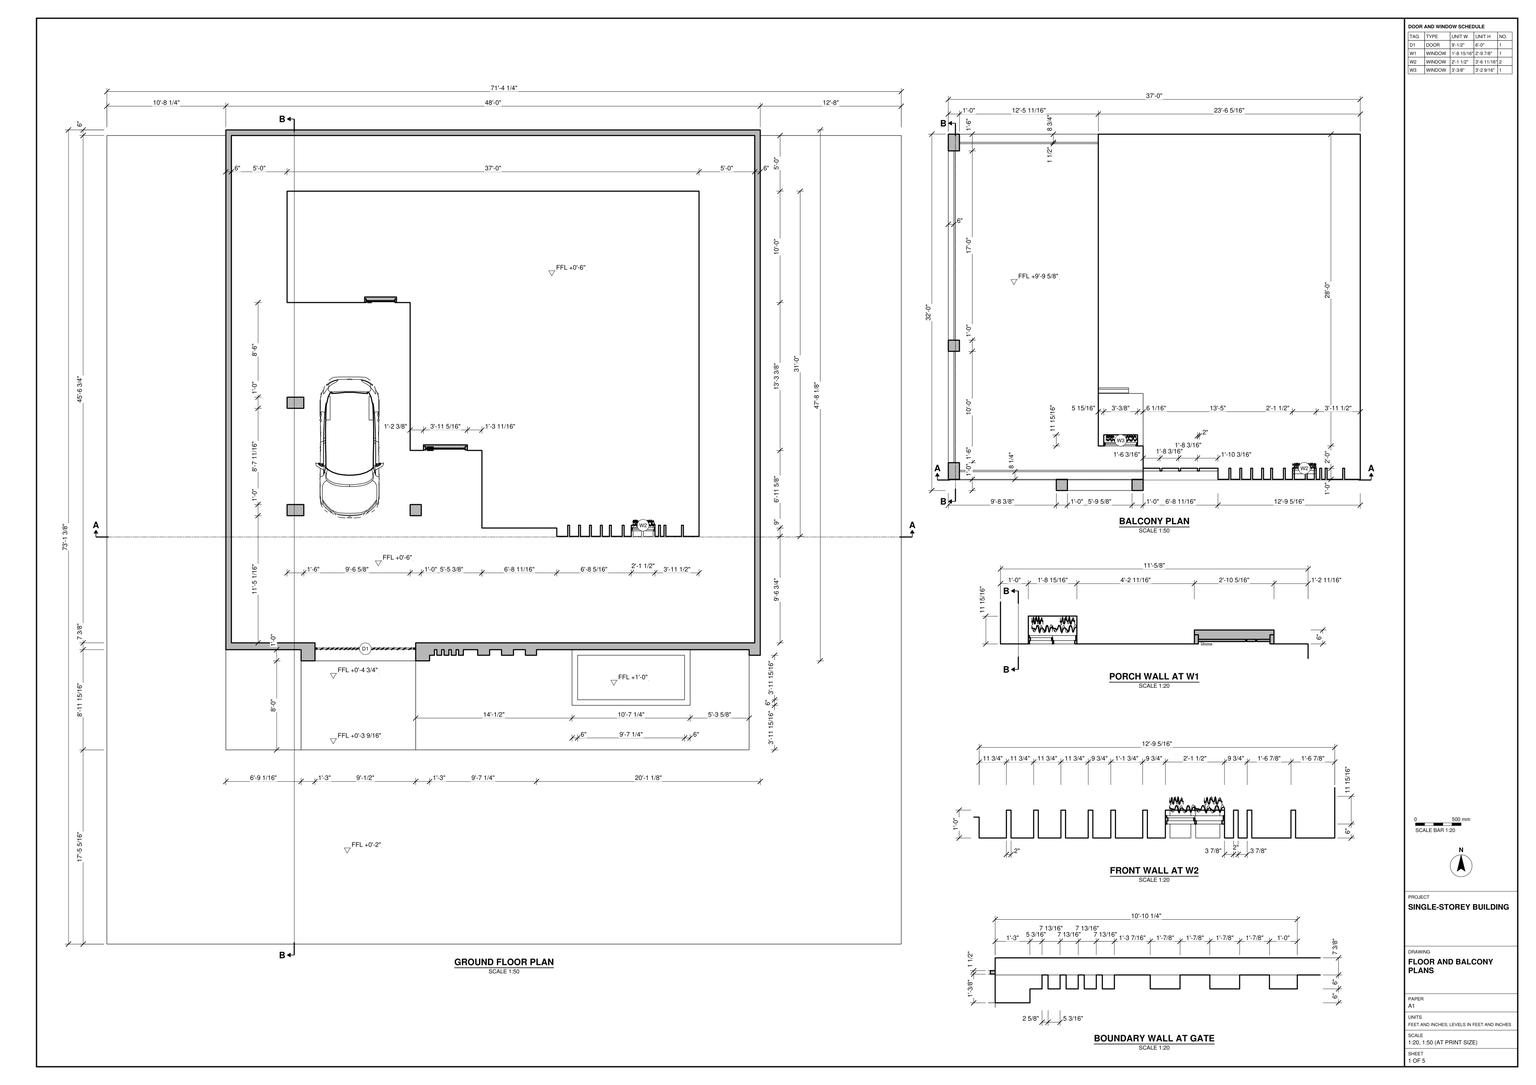
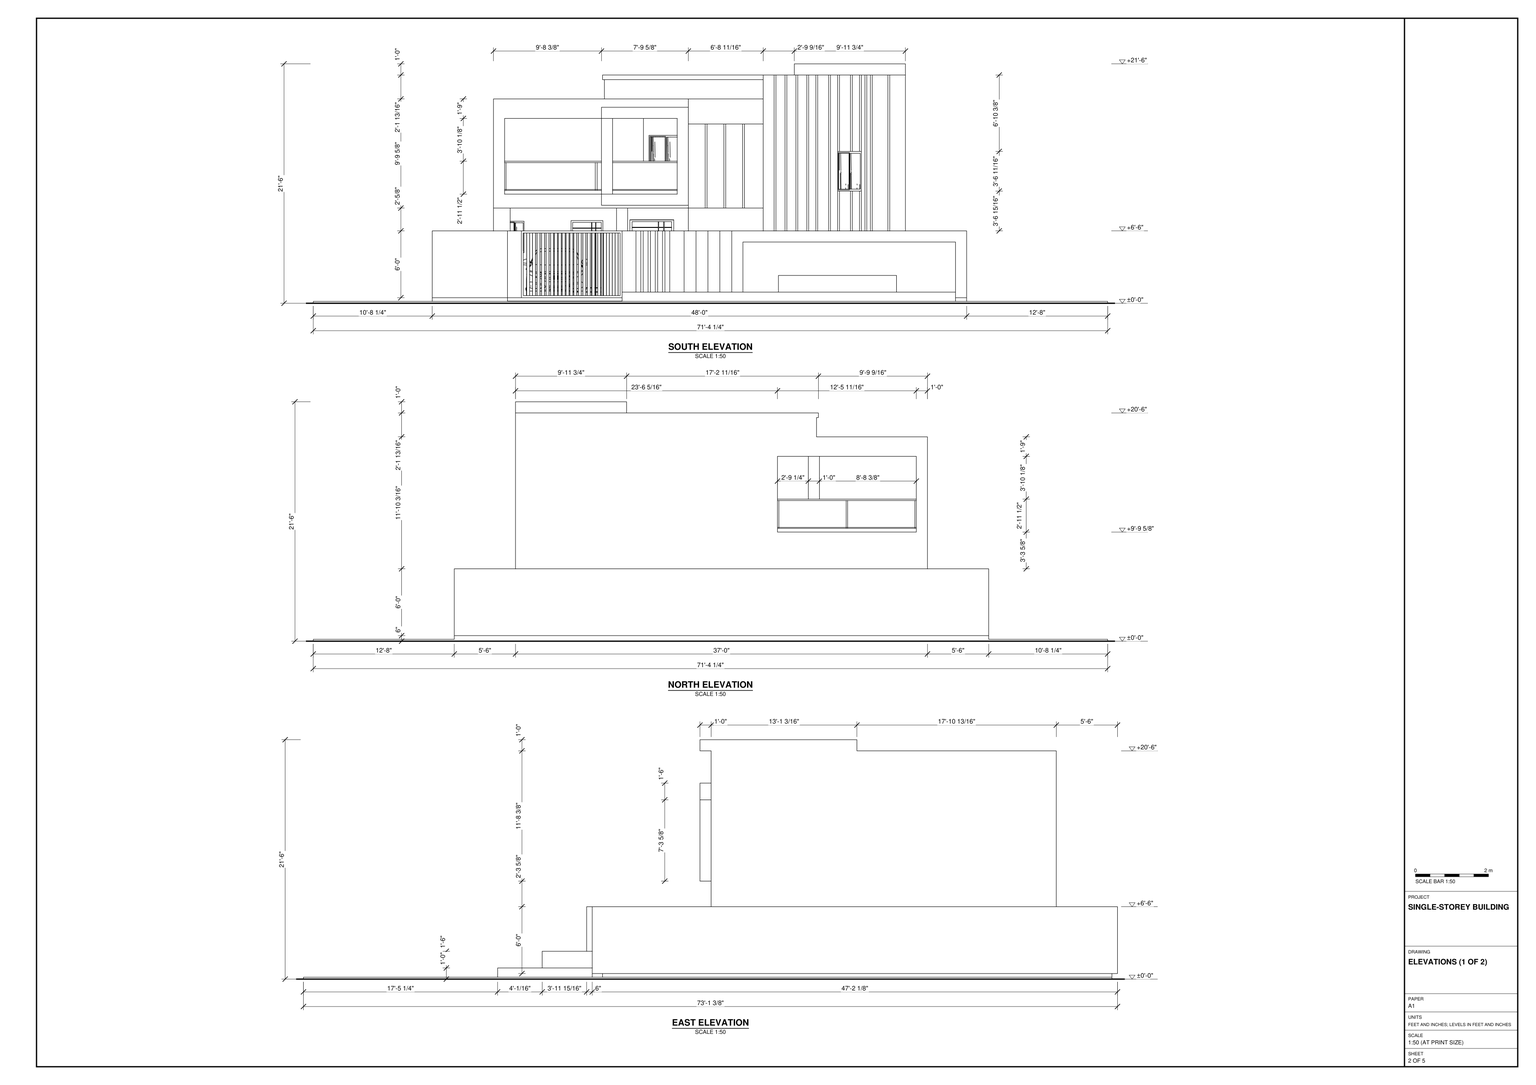
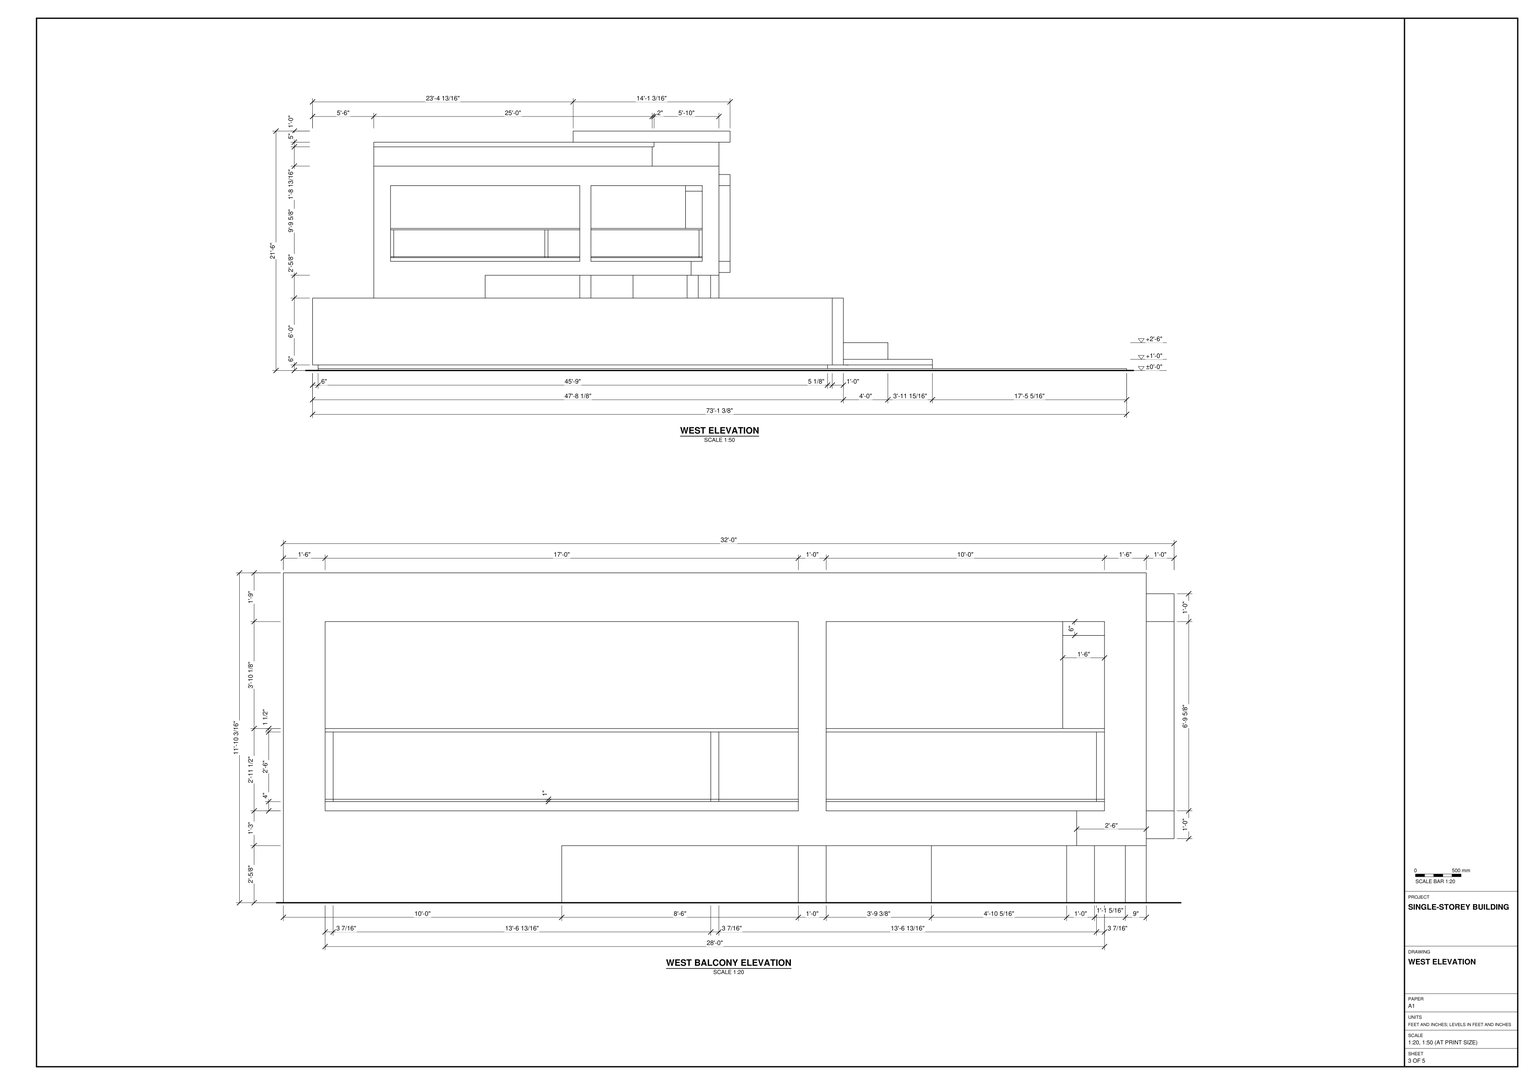
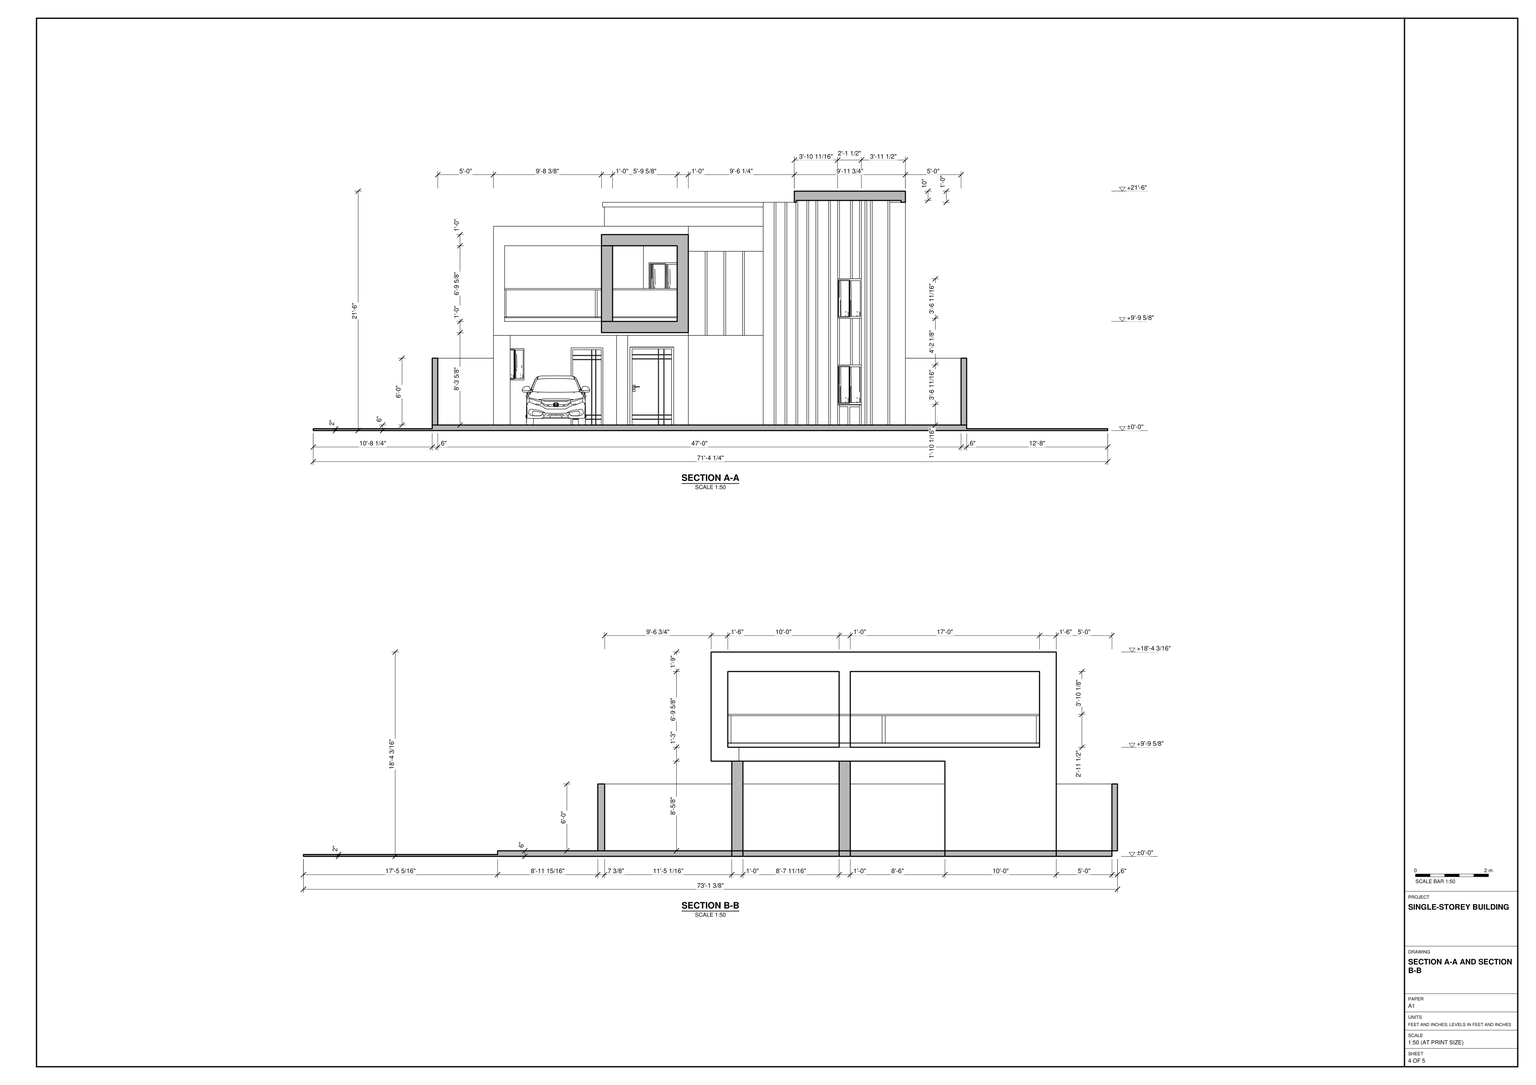
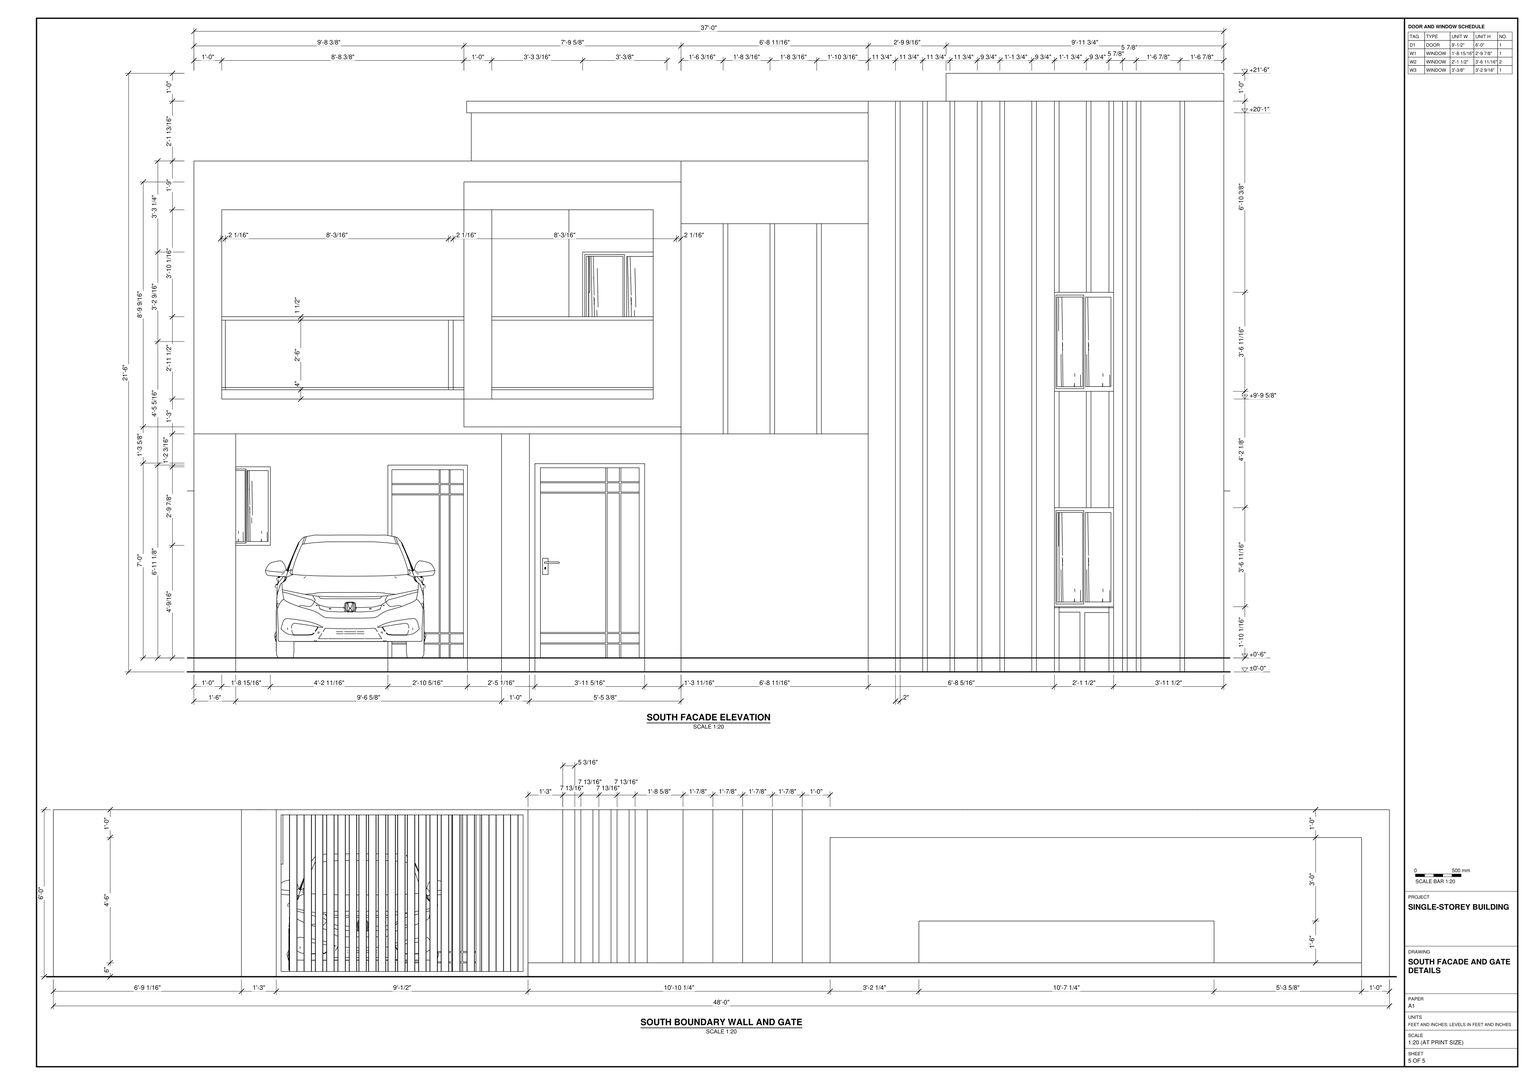
Build the house and its site in SketchUp from task_files/diagram_01.pdf. Work in feet and inches. Use ±0'-0" as the ground-floor datum. The complete model, including the site base, must measure 71'-4 1/4" east to west, 73'-1 3/8" north to south and 21'-6" high.

Lay out the boundary walls inside the site base, leaving the approach in front of the south gate. Follow the wall thicknesses in plan, including the 6" side boundary walls. Model the barred gate, the changing profile of the wall beside it and the low rectangular feature in front of the wall. Set the house back from the enclosure and follow the stepped ground-floor outline to form the recessed parking porch. Place the car under the balcony, in line with the gate.

Use the balcony plan and elevations to position the slab, supports, rectangular balcony frames and glass railing panels. Match the scheduled openings, the vertical fins around the front window and the stepped flat roof profile. Keep walls, slabs, roof elements and each furniture or joinery piece in separate groups or components, and use components for repeated parts. Decor and loose items, including the car, may be any suitable library components. Save one SketchUp model as output_files/single_storey_house_with_framed_balcony_and_gated_yard.skp.

# SketchUp Ruby script. Lengths in inches.
U = 1.inch
M = Sketchup.active_model
def pt(a) = Geom::Point3d.new(a.map { |v| v * U })
def face(e, loops, mat)
  f = e.add_face(loops[0].map { |a| pt(a) })
  loops[1..].each { |l| e.add_face(l.map { |a| pt(a) }).erase! }
  f.material = f.back_material = mat if mat
  f
end
# faces: each face lists its corners as indices into pts; further lists are holes
def faces(e, pts, list, mat = nil) = list.each { |f| face(e, (f[0].is_a?(Array) ? f : [f]).map { |l| l.map { |i| pts[i] } }, mat) }
# xy, xz, yz: faces in a plane at the given z, y or x. An outline is a flat list of corners, or four numbers for a rectangle; further outlines are holes
def ring(l) = l.size == 4 ? [[l[0], l[1]], [l[2], l[1]], [l[2], l[3]], [l[0], l[3]]] : l.each_slice(2).to_a
def flat(e, list, mat, &to3) = list.each { |f| face(e, (f[0].is_a?(Array) ? f : [f]).map { |l| ring(l).map { |u, v| to3.(u, v) } }, mat) }
def xy(e, z, list, mat = nil) = flat(e, list, mat) { |x, y| [x, y, z] }
def xz(e, y, list, mat = nil) = flat(e, list, mat) { |x, z| [x, y, z] }
def yz(e, x, list, mat = nil) = flat(e, list, mat) { |y, z| [x, y, z] }
def lines(e, pts, list) = list.each { |a, b| e.add_line(pt(pts[a]), pt(pts[b])) }
# prism: a flat outline (further loops are holes) pulled along v
def prism(e, loops, v, mat = nil)
  f = face(e, loops, mat); d = Geom::Vector3d.new(v.map { |x| x * U })
  f.pushpull(f.normal.samedirection?(d) ? d.length : -d.length)
end
def box(e, o, s, mat = nil) = prism(e, [[o, [o[0] + s[0], o[1], o[2]], [o[0] + s[0], o[1] + s[1], o[2]], [o[0], o[1] + s[1], o[2]]]], [0, 0, s[2]], mat)
def at(x, y, z, deg = 0) = Geom::Transformation.translation(pt([x, y, z])) * Geom::Transformation.rotation(ORIGIN, Z_AXIS, deg.degrees)
def axes(o, x, y, z) = Geom::Transformation.new([*x, 0, *y, 0, *z, 0, *pt(o).to_a, 1])
def part(name) = M.definitions.add(name)
# library, detail: a bought-in or finely detailed component or shape, given as its bounding box
def library(name, o, s) = part(name).tap { |d| box(d.entities, o, s) }
def detail(e, o, s) = box(e.add_group.entities, o, s)
def put(e, d, t, mat = nil) = e.add_instance(d, t).tap { |i| i.material = mat if mat }
def group(e, t, mat = nil) = e.add_group.tap { |g| g.transformation = t; g.material = mat if mat }.entities
root = M.entities
M.materials.add("Glass Railing Color").color = [198, 198, 198]
M.materials.add("Railing Glass").color = [63, 150, 137]
M.materials["Railing Glass"].alpha = 0.13
M.materials.add("[0053_Ivory]").color = [239, 239, 225]
M.materials.add("[0053_Ivory]1").color = [249, 249, 235]
M.materials.add("[0132_LightGray]").color = [169, 169, 169]
M.materials.add("[0135_DarkGray]").color = [81, 81, 81]
M.materials.add("[0136_Charcoal]").color = [48, 48, 48]
M.materials.add("[Concrete Block 8x8 Gray]").color = [210, 211, 206]
M.materials.add("[Stone Sandstone Ashlar Light]").color = [206, 178, 128]
M.materials.add("[Wood Veneer 01]").color = [120, 70, 37]
c1 = library("window",[15.03,5.78,0],[94.49,11.94,82.51])
c2 = part("Glass Rail Spacer")
box(c2.entities,[-0.5,-0.25,0],[1,0.5,1],"Glass Railing Color")
c3 = part("Group138\#1")
prism(c3.entities,[[[0.54,0,1.27],[0.38,0,1.39],[0.21,0,1.47],[0.01,0,1.5],[-0.18,0,1.48],[-0.37,0,1.41],[-0.52,0,1.29],[-0.64,0,1.13],[-0.72,0,0.96],[-0.75,0,0.76],[-0.73,0,0.57],[-0.66,0,0.38],[-0.54,0,0.23],[-0.38,0,0.11],[-0.21,0,0.03],[-0.01,0,0],[0.18,0,0.02],[0.37,0,0.09],[0.52,0,0.21],[0.64,0,0.37],[0.72,0,0.54],[0.75,0,0.74],[0.73,0,0.93],[0.66,0,1.12]]],[0,97,0],"Glass Railing Color")
c4 = part("Group141\#1")
prism(c4.entities,[[[0.25,0,5],[0.25,0,4],[-0.25,0,4],[-0.25,0,5],[-0.5,0,5],[-0.5,0,0],[0.5,0,0],[0.5,0,5]]],[0,97,0],"Glass Railing Color")
c5 = part("Group144\#1")
box(c5.entities,[-0.1875,0,0],[0.375,47,30],"Railing Glass")
c6 = part("Group147\#1")
box(c6.entities,[-0.1875,0,0],[0.375,47,30],"Railing Glass")
c7 = part("Glass Railing\#8")
put(c7.entities,c2,at(0,0,4))
put(c7.entities,c2,at(48,0,4))
put(c7.entities,c2,at(96,0,4))
put(c7.entities,c3,at(-0.5,0,34,-90))
put(c7.entities,c4,at(-0.5,0,0,-90))
put(c7.entities,c5,at(0.5,0,4,-90))
put(c7.entities,c6,at(48.5,0,4,-90))
c8 = library("Untitled (9)",[0,0,0],[36,4.39,84])
c9 = part("Group\#2")
box(c9.entities,[0,-0.5,0],[45,3,0.125])
c10 = part("Wade+gate+4.0")
p = [[1.5,-0.75,79.5],[1.5,-0.75,82.5]]
lines(c10.entities,p,[[0,1]])
g1 = group(c10.entities,at(0,-1.5,0),"[Wood Veneer 01]")
prism(g1,[[[48,0,6],[48,0,84],[0,0,84],[0,0,6]],[[46.5,0,82.5],[46.5,0,7.5],[1.5,0,7.5],[1.5,0,82.5]]],[0,1.5,0])
put(c10.entities,c9,axes([1.5,-1.46,78.96],[1,0,0],[0,0.64279,0.76604],[0,-0.76604,0.64279]),"[Wood Veneer 01]")
put(c10.entities,c9,axes([1.5,-1.46,74.46],[1,0,0],[0,0.64279,0.76604],[0,-0.76604,0.64279]),"[Wood Veneer 01]")
put(c10.entities,c9,axes([1.5,-1.46,69.96],[1,0,0],[0,0.64279,0.76604],[0,-0.76604,0.64279]),"[Wood Veneer 01]")
put(c10.entities,c9,axes([1.5,-1.46,65.46],[1,0,0],[0,0.64279,0.76604],[0,-0.76604,0.64279]),"[Wood Veneer 01]")
put(c10.entities,c9,axes([1.5,-1.46,60.96],[1,0,0],[0,0.64279,0.76604],[0,-0.76604,0.64279]),"[Wood Veneer 01]")
put(c10.entities,c9,axes([1.5,-1.46,57.46],[1,0,0],[0,0.64279,0.76604],[0,-0.76604,0.64279]),"[Wood Veneer 01]")
put(c10.entities,c9,axes([1.5,-1.46,53.96],[1,0,0],[0,0.64279,0.76604],[0,-0.76604,0.64279]),"[Wood Veneer 01]")
put(c10.entities,c9,axes([1.5,-1.46,50.46],[1,0,0],[0,0.64279,0.76604],[0,-0.76604,0.64279]),"[Wood Veneer 01]")
put(c10.entities,c9,axes([1.5,-1.46,46.96],[1,0,0],[0,0.64279,0.76604],[0,-0.76604,0.64279]),"[Wood Veneer 01]")
put(c10.entities,c9,axes([1.5,-1.46,43.96],[1,0,0],[0,0.64279,0.76604],[0,-0.76604,0.64279]),"[Wood Veneer 01]")
put(c10.entities,c9,axes([1.5,-1.46,40.96],[1,0,0],[0,0.64279,0.76604],[0,-0.76604,0.64279]),"[Wood Veneer 01]")
put(c10.entities,c9,axes([1.5,-1.46,37.96],[1,0,0],[0,0.64279,0.76604],[0,-0.76604,0.64279]),"[Wood Veneer 01]")
put(c10.entities,c9,axes([1.5,-1.46,34.96],[1,0,0],[0,0.64279,0.76604],[0,-0.76604,0.64279]),"[Wood Veneer 01]")
put(c10.entities,c9,axes([1.5,-1.46,31.96],[1,0,0],[0,0.64279,0.76604],[0,-0.76604,0.64279]),"[Wood Veneer 01]")
put(c10.entities,c9,axes([1.5,-1.46,28.96],[1,0,0],[0,0.64279,0.76604],[0,-0.76604,0.64279]),"[Wood Veneer 01]")
put(c10.entities,c9,axes([1.5,-1.46,25.46],[1,0,0],[0,0.64279,0.76604],[0,-0.76604,0.64279]),"[Wood Veneer 01]")
put(c10.entities,c9,axes([1.5,-1.46,21.96],[1,0,0],[0,0.64279,0.76604],[0,-0.76604,0.64279]),"[Wood Veneer 01]")
put(c10.entities,c9,axes([1.5,-1.46,18.46],[1,0,0],[0,0.64279,0.76604],[0,-0.76604,0.64279]),"[Wood Veneer 01]")
put(c10.entities,c9,axes([1.5,-1.46,14.96],[1,0,0],[0,0.64279,0.76604],[0,-0.76604,0.64279]),"[Wood Veneer 01]")
put(c10.entities,c9,axes([1.5,-1.46,10.46],[1,0,0],[0,0.64279,0.76604],[0,-0.76604,0.64279]),"[Wood Veneer 01]")
c11 = library("car\#1",[0.01,0.03,0.02],[18.76,39.97,12.32])
xy(root,-6,[[[0,0,856.25,871.375],[484.9375,439.375,484.9375,448.375,404.25,448.375,404.25,532,388.57,532,388.57,538,341.26,538,341.26,532,326.88,532,326.88,691.375,312.17,691.375,312.17,697.375,277.86,697.375,277.86,691.375,194.25,691.375,194.25,811.375,638.25,811.375,638.25,439.375,621.37,439.375,621.37,451.375,619.37,451.375,619.37,439.375,602.49,439.375,602.49,451.375,600.49,451.375,600.49,439.375,596.62,439.375,596.62,451.375,594.62,451.375,594.62,439.375,590.74,439.375,590.74,451.375,588.74,451.375,588.74,439.375,578.3,439.375,578.3,451.375,576.23,451.375,576.23,439.375,567.23,439.375,567.23,451.375,565.23,451.375,565.23,439.375,557.47,439.375,557.47,451.375,555.47,451.375,555.47,439.375,543.72,439.375,543.72,451.375,541.72,451.375,541.72,439.375,533.96,439.375,533.96,451.375,531.96,451.375,531.96,439.375,522.2,439.375,522.2,451.375,520.2,451.375,520.2,439.375,510.45,439.375,510.45,451.375,508.45,451.375,508.45,439.375,498.69,439.375,498.69,451.375,496.69,451.375,496.69,439.375],[194.25,461.6875,212.25,473.6875],[194.25,577.375,212.25,589.375],[326.88,461.6875,338.88,473.6875]],[484.9375,439.375,496.69,439.375,496.69,451.375,498.69,451.375,498.69,439.375,508.45,439.375,508.45,451.375,510.45,451.375,510.45,439.375,520.2,439.375,520.2,451.375,522.2,451.375,522.2,439.375,531.96,439.375,531.96,451.375,533.96,451.375,533.96,439.375,541.72,439.375,541.72,451.375,543.72,451.375,543.72,439.375,555.47,439.375,555.47,451.375,557.47,451.375,557.47,439.375,565.23,439.375,565.23,451.375,567.23,451.375,567.23,439.375,576.23,439.375,576.23,451.375,578.3,451.375,578.3,439.375,588.74,439.375,588.74,451.375,590.74,451.375,590.74,439.375,594.62,439.375,594.62,451.375,596.62,451.375,596.62,439.375,600.49,439.375,600.49,451.375,602.49,451.375,602.49,439.375,619.37,439.375,619.37,451.375,621.37,451.375,621.37,439.375,638.25,439.375,638.25,461.6875,404.25,461.6875,404.25,448.375,484.9375,448.375],[194.25,461.6875,212.25,473.6875],[404.25,461.6875,638.25,461.6875,638.25,811.375,194.25,811.375,194.25,691.375,277.86,691.375,277.86,697.375,312.17,697.375,312.17,691.375,326.88,691.375,326.88,532,341.26,532,341.26,538,388.57,538,388.57,532,404.25,532],[326.88,461.6875,338.88,473.6875],
  [194.25,577.375,212.25,589.375]])
xy(root,-4,[[209.36,209.28,332.875,209.3125,332.85,305.25,209.33,305.22],[332.875,209.3125,332.875,305.25,332.85,305.25]])
xy(root,-4,[[0,0,856.25,0,856.25,871.375,704.25,871.375,704.25,311.25,692.25,311.25,692.25,209.3125,332.875,209.3125,209.36,209.28,209.33,305.22,332.85,305.25,209.33,305.25,209.33,209.28,128.25,209.28,128.25,871.375,0,871.375]],"[Concrete Block 8x8 Gray]")
xy(root,0,[[209.33,305.25,209.33,317.25,128.25,317.25,128.25,322.375,134.25,322.375,134.25,324.625,224.33,324.625,224.33,305.25],[[224.33,305.25,332.85,305.25,332.85,324.625,698.25,324.625,698.25,871.375,134.25,871.375,134.25,324.625,224.33,324.625],[194.25,577.375,212.25,589.375],[194.25,461.6875,212.25,473.6875],[326.88,461.6875,338.88,473.6875]],[332.85,305.25,332.875,317.25],[332.875,305.25,332.875,317.25,353.05,317.25,353.05,311.25,347.85,311.25,347.85,305.25],[692.25,311.25,692.25,317.25,332.85,317.25,332.85,324.625,698.25,324.625,698.25,322.375,704.25,322.375,704.25,311.25],
  [355.65,311.25,360.85,317.25],[363.45,311.25,368.65,317.25],[371.25,311.25,376.45,317.25],[379.05,311.25,384.25,317.25],[399.7,311.25,412.55,317.25],
  [425.4,311.25,438.25,317.25],[451.1,311.25,463.1,317.25],[128.25,322.375,134.25,871.375],[698.25,322.375,704.25,871.375],[128.25,871.375,704.25,877.375]])
xy(root,0,[[194.25,461.6875,212.25,473.6875],[326.88,461.6875,338.88,473.6875],[194.25,577.375,212.25,589.375]],"[0135_DarkGray]")
xy(root,0,[[128.25,209.28,209.33,317.25]],"[Concrete Block 8x8 Gray]")
xy(root,6,[[507.39,263.28,622.64,311.25]],"[0053_Ivory]1")
xy(root,6,[[332.875,209.3125,692.25,209.3125,692.25,317.25,628.64,317.25,628.64,257.28,501.39,257.28,501.39,317.25,463.1,317.25,463.1,311.25,451.1,311.25,451.1,317.25,438.25,317.25,438.25,311.25,425.4,311.25,425.4,317.25,412.55,317.25,412.55,311.25,399.7,311.25,399.7,317.25,384.25,317.25,384.25,311.25,379.05,311.25,379.05,317.25,376.45,317.25,376.45,311.25,371.25,311.25,371.25,317.25,368.65,317.25,368.65,311.25,363.45,311.25,363.45,317.25,360.85,317.25,360.85,311.25,355.65,311.25,355.65,317.25,353.05,317.25,353.05,311.25,347.85,311.25,347.85,305.25,332.875,305.25]],"[Concrete Block 8x8 Gray]")
xy(root,19.5625,[[578.3,439.375,588.74,451.375]],"[Wood Veneer 01]")
xy(root,19.75,[[567.23,439.375,576.23,451.375]],"[Wood Veneer 01]")
xy(root,24,[[[501.39,257.28,628.64,317.25],[507.39,263.28,622.64,311.25]]],"[0053_Ivory]1")
xy(root,48.54,[[206.26,691.375,227.2,703.375]])
xy(root,60,[[463.1,311.25,692.25,317.25]],"[0135_DarkGray]")
xy(root,64.77,[[567.23,439.375,578.98,451.375]],"[0135_DarkGray]")
xy(root,64.77,[[580.98,439.375,588.74,451.375]],"[Wood Veneer 01]")
xy(root,72,[[209.33,305.25,224.33,305.25,224.33,324.625,134.25,324.625,134.25,871.375,698.25,871.375,698.25,324.625,332.85,324.625,332.85,305.25,347.85,305.25,347.85,311.25,353.05,311.25,353.05,317.25,355.65,317.25,355.65,311.25,360.85,311.25,360.85,317.25,363.45,317.25,363.45,311.25,368.65,311.25,368.65,317.25,371.25,317.25,371.25,311.25,376.45,311.25,376.45,317.25,379.05,317.25,379.05,311.25,384.25,311.25,384.25,317.25,399.7,317.25,399.7,311.25,412.55,311.25,412.55,317.25,425.4,317.25,425.4,311.25,438.25,311.25,438.25,317.25,451.1,317.25,451.1,311.25,704.25,311.25,704.25,877.375,128.25,877.375,128.25,317.25,209.33,317.25]],"[0053_Ivory]1")
xy(root,82.42,[[206.26,691.375,227.2,703.375]])
xy(root,83.125,[[277.86,691.375,312.17,697.375]])
xy(root,83.75,[[341.26,532,388.57,538]])
xy(root,96.6,[[404.25,448.375,422.42,451.375],[424.42,448.375,442.59,451.375],[444.59,448.375,462.77,451.375],[464.77,448.375,484.9375,451.375],[194.25,461.6875,212.25,473.6875],
  [194.25,577.375,212.25,589.375]])
xy(root,96.6,[[[194.25,439.375,194.25,461.6875,212.25,461.6875,212.25,473.6875,194.25,473.6875,194.25,577.375,212.25,577.375,212.25,589.375,194.25,589.375,194.25,691.375,326.88,691.375,326.88,532,404.25,532,404.25,439.375],[326.88,461.6875,338.88,473.6875]]],"[0053_Ivory]")
xy(root,99.6,[[310.65,427.375,404.25,439.375]],"[0135_DarkGray]")
xy(root,111.6,[[310.65,427.375,322.65,439.375]])
xy(root,111.6,[[206.25,439.375,404.25,439.375,404.25,475.375,355.91,475.375,355.91,811.375,206.25,811.375,206.25,793.375,194.25,793.375,194.25,589.375,206.25,589.375,206.25,577.375,194.25,577.375,194.25,457.375,206.25,457.375]],"[0053_Ivory]")
xy(root,111.6,[[322.65,427.375,392.25,439.375]],"[0135_DarkGray]")
xy(root,114.91,[[567.23,439.375,578.98,451.375]],"[0135_DarkGray]")
xy(root,114.91,[[580.98,439.375,588.74,451.375]],"[Wood Veneer 01]")
xy(root,136.41,[[361.82,475.375,398.19,487.375]])
xy(root,157.61,[[567.23,439.375,578.98,451.375]],"[0135_DarkGray]")
xy(root,157.61,[[580.98,439.375,588.74,451.375]],"[Wood Veneer 01]")
xy(root,174.97,[[361.82,475.375,398.19,487.375]])
xy(root,187.2,[[404.25,439.375,404.25,451.375,422.42,451.375,422.42,448.375,424.42,448.375,424.42,451.375,442.59,451.375,442.59,448.375,444.59,448.375,444.59,451.375,462.77,451.375,462.77,448.375,464.77,448.375,464.77,451.375,484.9375,451.375,484.9375,439.375]],"[0053_Ivory]")
xy(root,193.2,[[310.65,427.375,322.65,439.375]])
xy(root,193.2,[[[206.25,439.375,206.25,457.375,194.25,457.375,194.25,577.375,206.25,577.375,206.25,589.375,194.25,589.375,194.25,793.375,206.25,793.375,206.25,811.375,355.91,811.375,355.91,475.375,404.25,475.375,404.25,439.375],[206.46,481.3125,293.09,508.1875],[206.46,517.27,293.09,544.14],[206.46,553.22,293.09,580.1],[206.46,589.18,293.09,616.05],[206.46,625.13,293.09,652.01],[206.46,661.09,293.09,687.96],[206.46,733,293.09,759.875],[206.46,697.04,293.09,723.92]]],"[0053_Ivory]")
xy(root,193.2,[[322.65,427.375,392.25,439.375]],"[0135_DarkGray]")
xy(root,205.2,[[310.65,427.375,404.25,439.375]],"[0136_Charcoal]")
xy(root,214.2,[[[194.25,439.375,484.9375,439.375,484.9375,511.375,313.8125,511.375,313.8125,811.375,194.25,811.375],[206.46,481.3125,293.09,508.1875],[206.46,517.27,293.09,544.14],[206.46,553.22,293.09,580.1],[206.46,589.18,293.09,616.05],[206.46,625.13,293.09,652.01],[206.46,661.09,293.09,687.96],[206.46,733,293.09,759.875],[206.46,697.04,293.09,723.92]]],"[0053_Ivory]")
xy(root,235,[[311.8125,509.375,311.8125,811.375,313.8125,811.375,313.8125,511.375,484.9375,511.375,484.9375,509.375]],"[0135_DarkGray]")
xy(root,240,[[518.52,427.375,518.52,439.375,520.52,439.375,520.52,429.375,638.25,429.375,638.25,427.375],[633.5,429.375,638.25,439.375]],"[0053_Ivory]")
xy(root,240,[[484.9375,439.375,496.69,439.375,496.69,451.375,498.69,451.375,498.69,439.375,508.45,439.375,508.45,451.375,510.45,451.375,510.45,439.375,518.52,439.375,518.52,596.54,638.25,596.54,638.25,811.375,311.8125,811.375,311.8125,509.375,484.9375,509.375]],"[0135_DarkGray]")
xy(root,242,[[520.52,429.375,520.52,439.375,520.2,439.375,520.2,451.375,522.2,451.375,522.2,439.375,531.96,439.375,531.96,451.375,533.96,451.375,533.96,439.375,541.72,439.375,541.72,451.375,543.72,451.375,543.72,439.375,555.47,439.375,555.47,451.375,557.47,451.375,557.47,439.375,565.23,439.375,565.23,451.375,567.23,451.375,567.23,439.375,578.98,439.375,578.98,451.375,580.98,451.375,580.98,439.375,588.74,439.375,588.74,451.375,590.74,451.375,590.74,439.375,594.62,439.375,594.62,451.375,596.62,451.375,596.62,439.375,600.49,439.375,600.49,451.375,602.49,451.375,602.49,439.375,633.5,439.375,633.5,429.375],[619.37,439.375,621.37,451.375]],"[0053_Ivory]")
xy(root,252,[[518.52,427.375,638.25,596.54]],"[0053_Ivory]")
xz(root,0,[[0,-6,856.25,-4]])
xz(root,209.28,[[128.25,-4,209.33,0]],"[Concrete Block 8x8 Gray]")
xz(root,209.3125,[[332.875,-4,692.25,6,332.875,-3.67]])
xz(root,209.3125,[[332.875,-4,692.25,-4,692.25,6],[332.875,-3.67,692.25,6,332.875,6]],"[Concrete Block 8x8 Gray]")
xz(root,257.28,[[501.39,6,628.64,24]],"[0053_Ivory]1")
xz(root,263.28,[[507.39,6,622.64,24]],"[0053_Ivory]1")
xz(root,305.25,[[209.33,-4,224.33,0],[224.33,-4,332.85,0],[332.85,-4,332.875,0],[332.875,0,347.85,6]])
xz(root,305.25,[[209.33,0,224.33,72]],"[0053_Ivory]1")
xz(root,305.25,[[332.85,0,332.875,0,332.875,6,347.85,6,347.85,72,332.85,72]],"[Wood Veneer 01]")
xz(root,311.25,[[692.25,-4,704.25,0],[347.85,0,353.05,6],[355.65,0,360.85,6],[363.45,0,368.65,6],[371.25,0,376.45,6],
  [379.05,0,384.25,6],[399.7,0,412.55,6],[425.4,0,438.25,6],[451.1,0,463.1,6]])
xz(root,311.25,[[507.39,6,622.64,24]],"[0053_Ivory]1")
xz(root,311.25,[[692.25,0,704.25,0,704.25,72,451.1,72,451.1,6,463.1,6,463.1,60,692.25,60],[399.7,6,412.55,72],[425.4,6,438.25,72]],"[0135_DarkGray]")
xz(root,311.25,[[347.85,6,353.05,72],[355.65,6,360.85,72],[363.45,6,368.65,72],[371.25,6,376.45,72],[379.05,6,384.25,72]],"[Wood Veneer 01]")
xz(root,317.25,[[353.05,0,355.65,6],[360.85,0,363.45,6],[368.65,0,371.25,6],[376.45,0,379.05,6],[384.25,0,386.85,6],
  [386.85,0,399.7,6],[412.55,0,425.4,6],[438.25,0,451.1,6],[463.1,0,692.25,0,692.25,6,628.64,6,628.64,24,501.39,24,501.39,6,463.1,6]])
xz(root,317.25,[[128.25,0,209.33,72],[384.25,6,399.7,72],[412.55,6,425.4,72],[438.25,6,451.1,72]],"[0053_Ivory]1")
xz(root,317.25,[[463.1,6,501.39,6,501.39,24,628.64,24,628.64,6,692.25,6,692.25,60,463.1,60]],"[0132_LightGray]")
xz(root,317.25,[[353.05,6,355.65,72],[360.85,6,363.45,72],[368.65,6,371.25,72],[376.45,6,379.05,72]],"[Wood Veneer 01]")
xz(root,324.625,[[134.25,0,224.33,72],[332.85,0,698.25,72]])
xz(root,427.375,[[518.52,240,638.25,252]],"[0053_Ivory]")
xz(root,427.375,[[310.65,99.6,404.25,99.6,404.25,205.2,310.65,205.2,310.65,193.2,392.25,193.2,392.25,111.6,310.65,111.6],[310.65,111.6,322.65,193.2]],"[0135_DarkGray]")
xz(root,429.375,[[520.52,240,633.5,242]],"[0053_Ivory]")
xz(root,439.375,[[310.65,99.6,404.25,111.6],[310.65,193.2,404.25,205.2],[520.2,240,520.52,242]])
xz(root,439.375,[[621.37,0,638.25,240],[194.25,96.6,404.25,96.6,404.25,99.6,310.65,99.6,310.65,111.6,206.25,111.6,206.25,193.2,310.65,193.2,310.65,205.2,404.25,205.2,404.25,214.2,194.25,214.2],[404.25,187.2,484.9375,214.2],[621.37,240,633.5,242]],"[0053_Ivory]")
xz(root,439.375,[[621.37,-6,638.25,0]],"[0053_Ivory]1")
xz(root,439.375,[[484.9375,-6,496.69,0],[498.69,-6,508.45,0],[510.45,-6,520.2,0],[522.2,-6,531.96,0],[533.96,-6,541.72,0],
  [543.72,-6,555.47,0],[602.49,-6,619.37,0],[484.9375,0,496.69,240],[498.69,0,508.45,240],[510.45,0,520.2,240],
  [522.2,0,531.96,242],[533.96,0,541.72,242],[543.72,0,555.47,242],[602.49,0,619.37,242],[567.23,64.77,578.98,114.91],
  [310.65,111.6,322.65,193.2],[392.25,111.6,404.25,193.2],[567.23,157.61,578.98,242]],"[0135_DarkGray]")
xz(root,439.375,[[557.47,-6,565.23,0],[567.23,-6,576.23,0],[578.3,-6,588.74,0],[590.74,-6,594.62,0],[596.62,-6,600.49,0],
  [557.47,0,565.23,242],[567.23,0,576.23,19.75],[578.3,0,588.74,19.5625],[590.74,0,594.62,242],[596.62,0,600.49,242],
  [580.98,64.77,588.74,114.91],[580.98,157.61,588.74,242]],"[Wood Veneer 01]")
xz(root,448.375,[[422.42,96.6,424.42,187.2],[442.59,96.6,444.59,187.2],[462.77,96.6,464.77,187.2]])
xz(root,448.375,[[404.25,-6,484.9375,96.6]],"[Stone Sandstone Ashlar Light]")
xz(root,451.375,[[565.23,21.65,567.23,64.77],[567.23,21.65,588.74,64.77],[588.74,21.65,590.74,64.77],[565.23,114.91,590.74,157.61]])
xz(root,451.375,[[619.37,0,621.37,242]],"[0053_Ivory]")
xz(root,451.375,[[496.69,-6,498.69,0],[508.45,-6,510.45,0],[520.2,-6,522.2,0],[531.96,-6,533.96,0],[541.72,-6,543.72,0],
  [555.47,-6,557.47,0],[619.37,-6,621.37,0],[496.69,0,498.69,240],[508.45,0,510.45,240],[520.2,0,522.2,242],
  [531.96,0,533.96,242],[541.72,0,543.72,242],[555.47,0,557.47,242]],"[0135_DarkGray]")
xz(root,451.375,[[565.23,-6,567.23,0],[576.23,-6,578.3,0],[588.74,-6,590.74,0],[594.62,-6,596.62,0],[600.49,-6,602.49,0],
  [565.23,0,567.23,21.65],[576.23,0,578.3,0,578.3,19.5625,588.74,19.5625,588.74,21.65,567.23,21.65,567.23,19.75,576.23,19.75],[588.74,0,590.74,21.65],[594.62,0,596.62,242],[600.49,0,602.49,242],
  [565.23,64.77,567.23,114.91],[578.98,64.77,580.98,114.91],[588.74,64.77,590.74,114.91],[404.25,96.6,422.42,187.2],[424.42,96.6,442.59,187.2],
  [444.59,96.6,462.77,187.2],[464.77,96.6,484.9375,187.2],[565.23,157.61,567.23,242],[578.98,157.61,580.98,242],[588.74,157.61,590.74,242]],"[Wood Veneer 01]")
xz(root,457.375,[[194.25,111.6,206.25,193.2]])
xz(root,461.6875,[[194.25,-6,212.25,0],[326.88,-6,338.88,0],[194.25,0,212.25,96.6],[326.88,0,338.88,96.6]],"[0135_DarkGray]")
xz(root,473.6875,[[326.88,-6,338.88,0]])
xz(root,473.6875,[[194.25,-6,212.25,0],[194.25,0,212.25,96.6],[326.88,0,338.88,96.6]],"[0135_DarkGray]")
xz(root,475.375,[[[355.91,111.6,404.25,193.2],[361.82,136.41,398.19,174.97]]],"[0053_Ivory]")
xz(root,481.3125,[[206.46,193.2,293.09,214.2]],"[0053_Ivory]")
xz(root,487.375,[[361.82,136.41,398.19,174.97]])
xz(root,508.1875,[[206.46,193.2,293.09,214.2]],"[0053_Ivory]")
xz(root,509.375,[[311.8125,235,484.9375,240]],"[0135_DarkGray]")
xz(root,511.375,[[313.8125,214.2,484.9375,235]],"[0135_DarkGray]")
xz(root,517.27,[[206.46,193.2,293.09,214.2]],"[0053_Ivory]")
xz(root,532,[[326.88,0,341.26,0,341.26,83.75,388.57,83.75,388.57,0,404.25,0,404.25,96.6,326.88,96.6]],"[0053_Ivory]")
xz(root,532,[[326.88,-6,341.26,0],[388.57,-6,404.25,0]],"[0053_Ivory]1")
xz(root,538,[[341.26,0,388.57,83.75]])
xz(root,538,[[341.26,-6,388.57,0]],"[Wood Veneer 01]")
xz(root,544.14,[[206.46,193.2,293.09,214.2]],"[0053_Ivory]")
xz(root,553.22,[[206.46,193.2,293.09,214.2]],"[0053_Ivory]")
xz(root,577.375,[[194.25,111.6,206.25,193.2]],"[0053_Ivory]")
xz(root,577.375,[[194.25,-6,212.25,0],[194.25,0,212.25,96.6]],"[0135_DarkGray]")
xz(root,580.1,[[206.46,193.2,293.09,214.2]],"[0053_Ivory]")
xz(root,589.18,[[206.46,193.2,293.09,214.2]],"[0053_Ivory]")
xz(root,589.375,[[194.25,111.6,206.25,193.2]],"[0053_Ivory]")
xz(root,589.375,[[194.25,-6,212.25,0],[194.25,0,212.25,96.6]],"[0135_DarkGray]")
xz(root,596.54,[[518.52,240,638.25,252]],"[0053_Ivory]")
xz(root,616.05,[[206.46,193.2,293.09,214.2]],"[0053_Ivory]")
xz(root,625.13,[[206.46,193.2,293.09,214.2]],"[0053_Ivory]")
xz(root,652.01,[[206.46,193.2,293.09,214.2]],"[0053_Ivory]")
xz(root,661.09,[[206.46,193.2,293.09,214.2]],"[0053_Ivory]")
xz(root,687.96,[[206.46,193.2,293.09,214.2]],"[0053_Ivory]")
xz(root,691.375,[[[194.25,0,277.86,0,277.86,83.125,312.17,83.125,312.17,0,326.88,0,326.88,96.6,194.25,96.6],[206.26,48.54,227.2,82.42]]],"[0053_Ivory]")
xz(root,691.375,[[194.25,-6,277.86,0],[312.17,-6,326.88,0]],"[0053_Ivory]1")
xz(root,697.04,[[206.46,193.2,293.09,214.2]],"[0053_Ivory]")
xz(root,697.375,[[277.86,0,312.17,83.125]])
xz(root,697.375,[[277.86,-6,312.17,0]],"[Wood Veneer 01]")
xz(root,703.375,[[206.26,48.54,227.2,82.42]])
xz(root,723.92,[[206.46,193.2,293.09,214.2]],"[0053_Ivory]")
xz(root,733,[[206.46,193.2,293.09,214.2]],"[0053_Ivory]")
xz(root,759.875,[[206.46,193.2,293.09,214.2]],"[0053_Ivory]")
xz(root,793.375,[[194.25,111.6,206.25,193.2]],"[0053_Ivory]")
xz(root,811.375,[[[194.25,0,194.25,214.2,313.8125,214.2,313.8125,235,311.8125,235,311.8125,240,638.25,240,638.25,0],[206.25,111.6,355.91,193.2]]],"[0053_Ivory]")
xz(root,811.375,[[194.25,-6,638.25,0]],"[0053_Ivory]1")
xz(root,871.375,[[0,-6,0,-4,128.25,-4,128.25,0,704.25,0,704.25,-4,856.25,-4,856.25,-6],[134.25,0,698.25,72]],"[0053_Ivory]1")
xz(root,877.375,[[128.25,0,704.25,72]])
yz(root,0,[[0,-6,871.375,-4]])
yz(root,128.25,[[209.28,-4,322.375,0],[322.375,-4,871.375,0]])
yz(root,128.25,[[317.25,0,877.375,72]],"[0053_Ivory]1")
yz(root,134.25,[[324.625,0,871.375,72]])
yz(root,194.25,[[[691.375,0,691.375,96.6,469.375,96.6,469.375,111.6,577.375,111.6,577.375,193.2,457.375,193.2,457.375,111.6,469.375,111.6,469.375,96.6,439.375,96.6,439.375,214.2,811.375,214.2,811.375,0],[589.375,111.6,793.375,193.2]]],"[0053_Ivory]")
yz(root,194.25,[[691.375,-6,811.375,0]],"[0053_Ivory]1")
yz(root,194.25,[[461.6875,-6,473.6875,0],[577.375,-6,589.375,0],[461.6875,0,473.6875,96.6],[577.375,0,589.375,96.6]],"[0135_DarkGray]")
yz(root,206.25,[[439.375,111.6,457.375,193.2],[577.375,111.6,589.375,193.2],[793.375,111.6,811.375,193.2]])
yz(root,206.26,[[691.375,48.54,703.375,82.42]])
yz(root,206.46,[[481.3125,193.2,508.1875,214.2],[517.27,193.2,544.14,214.2],[553.22,193.2,580.1,214.2],[589.18,193.2,616.05,214.2],[625.13,193.2,652.01,214.2],
  [661.09,193.2,687.96,214.2],[697.04,193.2,723.92,214.2],[733,193.2,759.875,214.2]],"[0053_Ivory]")
yz(root,209.33,[[209.28,-4,305.22,0],[305.22,-4,305.25,0]])
yz(root,209.33,[[305.25,0,317.25,72]],"[0053_Ivory]1")
yz(root,212.25,[[461.6875,-6,473.6875,0],[577.375,-6,589.375,0],[461.6875,0,473.6875,96.6],[577.375,0,589.375,96.6]],"[0135_DarkGray]")
yz(root,224.33,[[305.25,0,324.625,72]],"[0053_Ivory]1")
yz(root,227.2,[[691.375,48.54,703.375,82.42]])
yz(root,277.86,[[691.375,0,697.375,83.125]])
yz(root,277.86,[[691.375,-6,697.375,0]],"[Wood Veneer 01]")
yz(root,293.09,[[481.3125,193.2,508.1875,214.2],[517.27,193.2,544.14,214.2],[553.22,193.2,580.1,214.2],[589.18,193.2,616.05,214.2],[625.13,193.2,652.01,214.2],
  [661.09,193.2,687.96,214.2],[697.04,193.2,723.92,214.2],[733,193.2,759.875,214.2]],"[0053_Ivory]")
yz(root,310.65,[[427.375,99.6,439.375,111.6]],"[0135_DarkGray]")
yz(root,310.65,[[427.375,111.6,439.375,193.2],[427.375,193.2,439.375,205.2]],"[0136_Charcoal]")
yz(root,311.8125,[[509.375,235,811.375,240]],"[0135_DarkGray]")
yz(root,312.17,[[691.375,0,697.375,83.125]])
yz(root,312.17,[[691.375,-6,697.375,0]],"[Wood Veneer 01]")
yz(root,313.8125,[[511.375,214.2,811.375,235]],"[0135_DarkGray]")
yz(root,322.65,[[427.375,111.6,439.375,193.2]],"[0135_DarkGray]")
yz(root,326.88,[[532,0,691.375,96.6]],"[0053_Ivory]")
yz(root,326.88,[[532,-6,691.375,0]],"[0053_Ivory]1")
yz(root,326.88,[[461.6875,-6,473.6875,0],[461.6875,0,473.6875,96.6]],"[0135_DarkGray]")
yz(root,332.85,[[305.25,0,324.625,72]],"[Wood Veneer 01]")
yz(root,332.875,[[209.3125,-3.67,209.3125,6,257.28,6],[209.3125,-3.67,257.28,6,305.25,0],[305.25,0,257.28,6,305.25,6]])
yz(root,338.88,[[461.6875,-6,473.6875,0],[461.6875,0,473.6875,96.6]],"[0135_DarkGray]")
yz(root,341.26,[[532,0,538,83.75]])
yz(root,341.26,[[532,-6,538,0]],"[Wood Veneer 01]")
yz(root,347.85,[[305.25,0,311.25,6]])
yz(root,347.85,[[305.25,6,311.25,72]],"[Wood Veneer 01]")
yz(root,353.05,[[311.25,0,317.25,6]])
yz(root,353.05,[[311.25,6,317.25,72]],"[Wood Veneer 01]")
yz(root,355.65,[[311.25,0,317.25,6]])
yz(root,355.65,[[311.25,6,317.25,72]],"[Wood Veneer 01]")
yz(root,355.91,[[475.375,111.6,811.375,193.2]],"[0053_Ivory]")
yz(root,360.85,[[311.25,0,317.25,6]])
yz(root,360.85,[[311.25,6,317.25,72]],"[Wood Veneer 01]")
yz(root,361.82,[[475.375,136.41,487.375,174.97]])
yz(root,363.45,[[311.25,0,317.25,6]])
yz(root,363.45,[[311.25,6,317.25,72]],"[Wood Veneer 01]")
yz(root,368.65,[[311.25,0,317.25,6]])
yz(root,368.65,[[311.25,6,317.25,72]],"[Wood Veneer 01]")
yz(root,371.25,[[311.25,0,317.25,6]])
yz(root,371.25,[[311.25,6,317.25,72]],"[Wood Veneer 01]")
yz(root,376.45,[[311.25,0,317.25,6]])
yz(root,376.45,[[311.25,6,317.25,72]],"[Wood Veneer 01]")
yz(root,379.05,[[311.25,0,317.25,6]])
yz(root,379.05,[[311.25,6,317.25,72]],"[Wood Veneer 01]")
yz(root,384.25,[[311.25,0,317.25,6]])
yz(root,384.25,[[311.25,6,317.25,72]],"[Wood Veneer 01]")
yz(root,388.57,[[532,0,538,83.75]])
yz(root,388.57,[[532,-6,538,0]],"[Wood Veneer 01]")
yz(root,392.25,[[427.375,111.6,439.375,193.2]],"[0135_DarkGray]")
yz(root,398.19,[[475.375,136.41,487.375,174.97]])
yz(root,399.7,[[311.25,0,317.25,6]])
yz(root,399.7,[[311.25,6,317.25,72]],"[0135_DarkGray]")
yz(root,404.25,[[439.375,96.6,451.375,111.6]])
yz(root,404.25,[[439.375,111.6,451.375,187.2],[451.375,111.6,475.375,187.2],[439.375,187.2,475.375,193.2]],"[0053_Ivory]")
yz(root,404.25,[[427.375,99.6,439.375,187.2],[427.375,187.2,439.375,205.2]],"[0135_DarkGray]")
yz(root,404.25,[[448.375,-6,532,96.6]],"[Stone Sandstone Ashlar Light]")
yz(root,412.55,[[311.25,0,317.25,6]])
yz(root,412.55,[[311.25,6,317.25,72]],"[0135_DarkGray]")
yz(root,422.42,[[448.375,96.6,451.375,187.2]])
yz(root,424.42,[[448.375,96.6,451.375,187.2]])
yz(root,425.4,[[311.25,0,317.25,6]])
yz(root,425.4,[[311.25,6,317.25,72]],"[0135_DarkGray]")
yz(root,438.25,[[311.25,0,317.25,6]])
yz(root,438.25,[[311.25,6,317.25,72]],"[0135_DarkGray]")
yz(root,442.59,[[448.375,96.6,451.375,187.2]])
yz(root,444.59,[[448.375,96.6,451.375,187.2]])
yz(root,451.1,[[311.25,0,317.25,6]])
yz(root,451.1,[[311.25,6,317.25,72]],"[0135_DarkGray]")
yz(root,462.77,[[448.375,96.6,451.375,187.2]])
yz(root,463.1,[[311.25,0,317.25,6]])
yz(root,463.1,[[311.25,6,317.25,60]],"[0135_DarkGray]")
yz(root,464.77,[[448.375,96.6,451.375,187.2]])
yz(root,484.9375,[[439.375,-6,448.375,0],[439.375,0,439.375,187.2,451.375,187.2,451.375,96.6,448.375,96.6,448.375,0],[439.375,214.2,439.375,240,509.375,240,509.375,235,511.375,235,511.375,214.2]],"[0135_DarkGray]")
yz(root,496.69,[[439.375,-6,451.375,0],[439.375,0,451.375,240]],"[0135_DarkGray]")
yz(root,498.69,[[439.375,-6,451.375,0],[439.375,0,451.375,240]],"[0135_DarkGray]")
yz(root,501.39,[[257.28,6,317.25,24]],"[0053_Ivory]1")
yz(root,507.39,[[263.28,6,311.25,24]],"[0053_Ivory]1")
yz(root,508.45,[[439.375,-6,451.375,0],[439.375,0,451.375,240]],"[0135_DarkGray]")
yz(root,510.45,[[439.375,-6,451.375,0],[439.375,0,451.375,240]],"[0135_DarkGray]")
yz(root,518.52,[[427.375,240,596.54,252]],"[0053_Ivory]")
yz(root,520.2,[[439.375,-6,451.375,0],[439.375,0,451.375,242]],"[0135_DarkGray]")
yz(root,520.52,[[429.375,240,439.375,242]])
yz(root,522.2,[[439.375,-6,451.375,0],[439.375,0,451.375,242]],"[0135_DarkGray]")
yz(root,531.96,[[439.375,-6,451.375,0],[439.375,0,451.375,242]],"[0135_DarkGray]")
yz(root,533.96,[[439.375,-6,451.375,0],[439.375,0,451.375,242]],"[0135_DarkGray]")
yz(root,541.72,[[439.375,-6,451.375,0],[439.375,0,451.375,242]],"[0135_DarkGray]")
yz(root,543.72,[[439.375,-6,451.375,0],[439.375,0,451.375,242]],"[0135_DarkGray]")
yz(root,555.47,[[439.375,-6,451.375,0],[439.375,0,451.375,242]],"[0135_DarkGray]")
yz(root,557.47,[[439.375,-6,451.375,0],[439.375,0,451.375,242]],"[Wood Veneer 01]")
yz(root,565.23,[[439.375,-6,451.375,0],[439.375,0,451.375,242]],"[Wood Veneer 01]")
yz(root,567.23,[[439.375,64.77,451.375,114.91],[439.375,157.61,451.375,242]],"[0135_DarkGray]")
yz(root,567.23,[[439.375,-6,451.375,0],[439.375,0,451.375,19.75]],"[Wood Veneer 01]")
yz(root,576.23,[[439.375,-6,451.375,0],[439.375,0,451.375,19.75]],"[Wood Veneer 01]")
yz(root,578.3,[[439.375,-6,451.375,0],[439.375,0,451.375,19.5625]],"[Wood Veneer 01]")
yz(root,578.98,[[439.375,64.77,451.375,114.91],[439.375,157.61,451.375,242]],"[0135_DarkGray]")
yz(root,580.98,[[439.375,64.77,451.375,114.91],[439.375,157.61,451.375,242]],"[Wood Veneer 01]")
yz(root,588.74,[[439.375,-6,451.375,0],[439.375,0,451.375,19.5625],[439.375,64.77,451.375,114.91],[439.375,157.61,451.375,242]],"[Wood Veneer 01]")
yz(root,590.74,[[439.375,-6,451.375,0],[439.375,0,451.375,242]],"[Wood Veneer 01]")
yz(root,594.62,[[439.375,-6,451.375,0],[439.375,0,451.375,242]],"[Wood Veneer 01]")
yz(root,596.62,[[439.375,-6,451.375,0],[439.375,0,451.375,242]],"[Wood Veneer 01]")
yz(root,600.49,[[439.375,-6,451.375,0],[439.375,0,451.375,242]],"[Wood Veneer 01]")
yz(root,602.49,[[439.375,-6,451.375,0],[439.375,0,451.375,242]],"[0135_DarkGray]")
yz(root,619.37,[[439.375,-6,451.375,0]],"[0053_Ivory]1")
yz(root,619.37,[[439.375,0,451.375,242]],"[0135_DarkGray]")
yz(root,621.37,[[439.375,0,451.375,242]],"[0053_Ivory]")
yz(root,621.37,[[439.375,-6,451.375,0]],"[0053_Ivory]1")
yz(root,622.64,[[263.28,6,311.25,24]],"[0053_Ivory]1")
yz(root,628.64,[[257.28,6,317.25,24]],"[0053_Ivory]1")
yz(root,633.5,[[429.375,240,439.375,242]],"[0053_Ivory]")
yz(root,638.25,[[439.375,0,811.375,0,811.375,240,596.54,240,596.54,252,427.375,252,427.375,240,439.375,240]],"[0053_Ivory]")
yz(root,638.25,[[439.375,-6,811.375,0]],"[0053_Ivory]1")
yz(root,692.25,[[209.3125,-4,311.25,6],[311.25,0,317.25,6]])
yz(root,692.25,[[311.25,6,317.25,60]],"[0135_DarkGray]")
yz(root,698.25,[[324.625,0,871.375,72]],"[0053_Ivory]1")
yz(root,704.25,[[311.25,-4,322.375,0],[322.375,-4,871.375,0]])
yz(root,704.25,[[311.25,0,877.375,72]],"[0053_Ivory]1")
yz(root,856.25,[[0,-6,871.375,-4]])
p = [[209.36,209.28,-4],[209.36,209.28,-3.67],[209.33,305.22,0],[209.33,305.22,-4],[332.875,209.3125,-4],[332.875,209.3125,-3.67],
  [332.85,305.25,0],[332.85,305.25,-4],[404.25,547.33,214.2],[313.8125,547.33,214.2],[404.25,583.29,214.2],[313.8125,583.29,214.2],
  [404.25,619.24,214.2],[313.8125,619.24,214.2],[404.25,655.2,214.2],[313.8125,655.2,214.2],[404.25,691.15,214.2],[313.8125,691.15,214.2],
  [404.25,727.11,214.2],[313.8125,727.11,214.2],[404.25,763.0625,214.2],[313.8125,763.0625,214.2],[518.52,439.375,242],[520.2,439.375,242]]
faces(root,p,[[0,1,2,3],[0,4,5],[5,1,0],[6,7,3,2]])
faces(root,p,[[5,6,2,1]],"[Concrete Block 8x8 Gray]")
lines(root,p,[[8,9],[10,11],[12,13],[14,15],[16,17],[18,19],[20,21],[22,23]])
put(root,c1,axes([403.98,493.09,136.41],[-0.38497,0,0],[0,-1,0],[0,0,0.46736]))
put(root,c1,axes([230.53,709.09,48.54],[-0.22159,0,0],[0,-1,0],[0,0,0.41058]))
put(root,c7,axes([206.77,448.375,111.6],[2.04639,0,0],[0,1,0],[0,0,1]))
put(root,c7,axes([201,791.64,111.6],[0,-3.46392,0],[1,0,0],[0,0,1]))
put(root,c7,axes([207.02,801.875,111.6],[1.54289,0,0],[0,1,0],[0,0,1]))
put(root,c8,axes([341.26,532,0],[1.31424,0,0],[0,1,0],[0,0,1]))
put(root,c8,axes([277.86,690.94,0],[0.95312,0,0],[0,1,0],[0,0,0.98958]))
put(root,c1,axes([594.8,463.09,114.91],[-0.27,0,0],[0,-1,0],[0,0,0.51753]))
put(root,c1,axes([594.8,463.09,22.07],[-0.27,0,0],[0,-1,0],[0,0,0.51753]))
put(root,c10,axes([215.98,319.125,72],[0,0,-1.5],[0,1,0],[1.39126,0,0]))
put(root,c11,axes([224.92,458.84,-0.07],[3.9078,0,0],[0,3.808,0],[0,0,4.3]))
